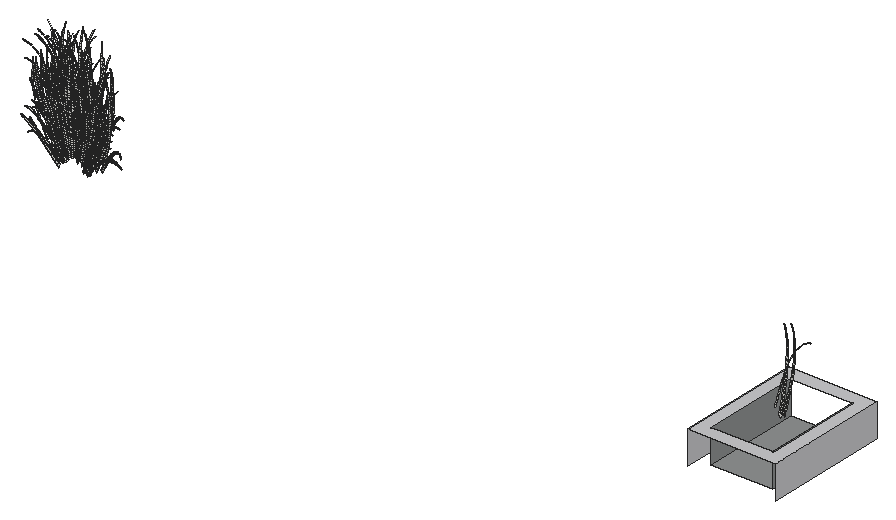
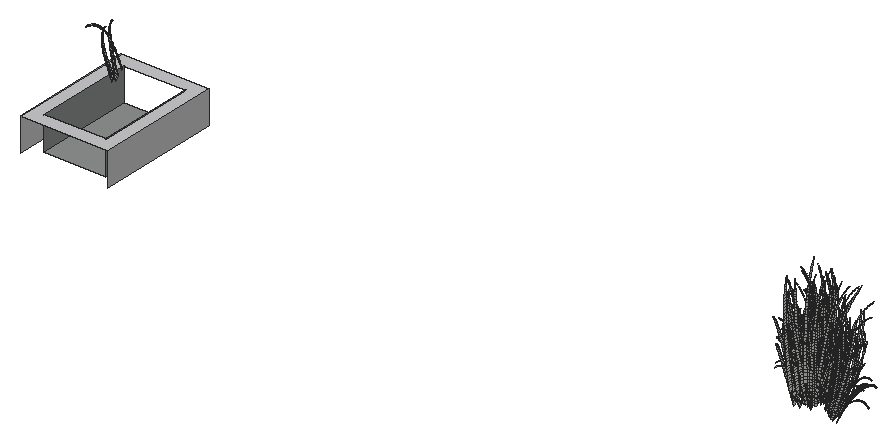
# SketchUp Ruby script. Lengths in inches.
U = 1.inch
M = Sketchup.active_model
def pt(a) = Geom::Point3d.new(a.map { |v| v * U })
def face(e, loops, mat)
  f = e.add_face(loops[0].map { |a| pt(a) })
  loops[1..].each { |l| e.add_face(l.map { |a| pt(a) }).erase! }
  f.material = f.back_material = mat if mat
  f
end
# faces: each face lists its corners as indices into pts; further lists are holes
def faces(e, pts, list, mat = nil) = list.each { |f| face(e, (f[0].is_a?(Array) ? f : [f]).map { |l| l.map { |i| pts[i] } }, mat) }
# xy, xz, yz: faces in a plane at the given z, y or x. An outline is a flat list of corners, or four numbers for a rectangle; further outlines are holes
def ring(l) = l.size == 4 ? [[l[0], l[1]], [l[2], l[1]], [l[2], l[3]], [l[0], l[3]]] : l.each_slice(2).to_a
def flat(e, list, mat, &to3) = list.each { |f| face(e, (f[0].is_a?(Array) ? f : [f]).map { |l| ring(l).map { |u, v| to3.(u, v) } }, mat) }
def xy(e, z, list, mat = nil) = flat(e, list, mat) { |x, y| [x, y, z] }
def xz(e, y, list, mat = nil) = flat(e, list, mat) { |x, z| [x, y, z] }
def yz(e, x, list, mat = nil) = flat(e, list, mat) { |y, z| [x, y, z] }
def lines(e, pts, list) = list.each { |a, b| e.add_line(pt(pts[a]), pt(pts[b])) }
# prism: a flat outline (further loops are holes) pulled along v
def prism(e, loops, v, mat = nil)
  f = face(e, loops, mat); d = Geom::Vector3d.new(v.map { |x| x * U })
  f.pushpull(f.normal.samedirection?(d) ? d.length : -d.length)
end
def box(e, o, s, mat = nil) = prism(e, [[o, [o[0] + s[0], o[1], o[2]], [o[0] + s[0], o[1] + s[1], o[2]], [o[0], o[1] + s[1], o[2]]]], [0, 0, s[2]], mat)
def at(x, y, z, deg = 0) = Geom::Transformation.translation(pt([x, y, z])) * Geom::Transformation.rotation(ORIGIN, Z_AXIS, deg.degrees)
def axes(o, x, y, z) = Geom::Transformation.new([*x, 0, *y, 0, *z, 0, *pt(o).to_a, 1])
def part(name) = M.definitions.add(name)
# library, detail: a bought-in or finely detailed component or shape, given as its bounding box
def library(name, o, s) = part(name).tap { |d| box(d.entities, o, s) }
def detail(e, o, s) = box(e.add_group.entities, o, s)
def put(e, d, t, mat = nil) = e.add_instance(d, t).tap { |i| i.material = mat if mat }
def group(e, t, mat = nil) = e.add_group.tap { |g| g.transformation = t; g.material = mat if mat }.entities
root = M.entities
M.materials.add("[Blacktop Old 02]").color = [143, 145, 145]
M.materials.add("[Polished Concrete New]").color = [200, 200, 203]
c1 = part("fur_instance\#8")
p = [[-0.25,1.49,0.03],[0.25,-1.49,-0.03],[0.44,-1.47,1.51],[-0.05,1.47,1.57],[0.65,-1.44,3.05],[0.16,1.45,3.11],
  [0.86,-1.42,4.59],[0.38,1.44,4.65],[1.1,-1.39,6.13],[0.62,1.43,6.18],[1.34,-1.35,7.66],[0.875,1.42,7.72],
  [1.6,-1.32,9.19],[1.14,1.41,9.25],[1.88,-1.28,10.72],[1.43,1.41,10.78],[2.18,-1.24,12.25],[1.73,1.41,12.3],
  [2.49,-1.19,13.77],[2.05,1.41,13.82],[2.83,-1.15,15.29],[2.4,1.41,15.34],[3.18,-1.09,16.8],[2.76,1.42,16.85],
  [3.56,-1.03,18.31],[3.14,1.43,18.35],[3.96,-0.97,19.81],[3.55,1.44,19.85],[4.38,-0.91,21.3],[3.99,1.46,21.35],
  [4.84,-0.83,22.78],[4.45,1.48,22.83],[5.32,-0.76,24.26],[4.93,1.51,24.31],[5.82,-0.67,25.73],[5.45,1.54,25.77],
  [6.36,-0.59,27.18],[6,1.57,27.23],[6.93,-0.49,28.625],[6.58,1.61,28.67],[7.54,-0.39,30.05],[7.19,1.66,30.1],
  [8.18,-0.28,31.47],[7.84,1.71,31.51],[8.85,-0.16,32.86],[8.53,1.77,32.9],[9.57,-0.04,34.24],[9.25,1.83,34.27],
  [10.32,0.09,35.59],[10.02,1.9,35.625],[11.12,0.23,36.92],[10.82,1.97,36.95],[11.95,0.38,38.22],[11.67,2.06,38.25],
  [12.84,0.54,39.49],[12.57,2.14,39.52],[13.76,0.71,40.73],[13.51,2.24,40.76],[14.73,0.89,41.93],[14.49,2.34,41.95],
  [15.75,1.08,43.09],[15.52,2.45,43.11],[16.82,1.28,44.2],[16.6,2.5625,44.23],[17.93,1.5,45.27],[17.73,2.68,45.29],
  [19.08,1.73,46.28],[18.9,2.81,46.3],[20.29,1.97,47.24],[20.125,2.93,47.26],[21.53,2.22,48.13],[21.39,3.0625,48.15],
  [22.82,2.5,48.96],[22.7,3.1875,48.98],[24.14,2.8125,49.72],[24.06,3.3,49.73],[25.48,3.27,50.41]]
faces(c1.entities,p,[[0,1,2,3],[3,2,4,5],[5,4,6,7],[7,6,8,9],[9,8,10,11],[11,10,12,13],[13,12,14,15],[15,14,16,17],
  [17,16,18,19],[19,18,20,21],[21,20,22,23],[23,22,24,25],[25,24,26,27],[27,26,28,29],[29,28,30,31],[31,30,32,33],
  [33,32,34,35],[35,34,36,37],[37,36,38,39],[39,38,40,41],[41,40,42,43],[43,42,44,45],[45,44,46,47],[47,46,48,49],
  [49,48,50,51],[51,50,52,53],[53,52,54,55],[55,54,56,57],[57,56,58,59],[59,58,60,61],[61,60,62,63],[63,62,64,65],
  [65,64,66,67],[67,66,68,69],[69,68,70,71],[71,70,72,73],[73,72,74,75],[75,74,76]])
xy(root,0,[[419.51,51.02,438.8125,82.15]],"[Blacktop Old 02]")
xy(root,10.375,[[[415.52,47.02,442.8125,86.15],[419.51,51.02,438.8125,82.15]]],"[Polished Concrete New]")
yz(root,415.52,[[47.02,0,86.15,10.375]],"[Polished Concrete New]")
yz(root,419.51,[[51.02,0,82.15,10.375]],"[Blacktop Old 02]")
yz(root,438.8125,[[51.02,0,82.15,10.375]],"[Blacktop Old 02]")
yz(root,442.8125,[[47.02,0,86.15,10.375]],"[Polished Concrete New]")
put(root,c1,axes([204.53,65.8125,2.49],[-0.13594,0.15084,-0.11164],[-0.0609,-0.07291,-0.33491],[-0.13519,-0.09407,0.27953]))
put(root,c1,axes([202.25,69.58,2.69],[0.13391,-0.00422,0.37894],[-0.02725,0.21287,-0.08205],[-0.17659,-0.01268,0.31548]))
put(root,c1,axes([204.92,66.53,3.77],[-0.14992,0.10635,-0.20855],[-0.03569,-0.13875,-0.18978],[-0.12006,-0.06524,0.33426]))
put(root,c1,axes([204.92,67.96,3.64],[-0.13947,0.07457,-0.26376],[-0.03048,-0.16347,-0.05841],[-0.12421,-0.01975,0.3263]))
put(root,c1,axes([204.95,66.7,2.23],[-0.11214,0.07357,-0.29467],[-0.00419,-0.1506,-0.10442],[-0.13991,-0.03543,0.25192]))
put(root,c1,axes([204.01,70.26,10.22],[-0.16722,-0.14584,-0.14657],[0.18274,-0.19209,0.09427],[-0.0816,-0.06233,0.55718]))
put(root,c1,axes([202.55,71.21,3.75],[0.10956,-0.18152,0.25882],[0.13509,0.11782,0.19082],[-0.14519,0.00192,0.39222]))
put(root,c1,axes([203.54,69.17,3.12],[0.07012,-0.18381,0.20265],[0.10518,0.07075,0.29594],[-0.16336,-0.01173,0.29184]))
put(root,c1,axes([203.42,66.95,2.47],[0.11177,0.01694,0.37048],[-0.08915,0.18926,-0.03147],[-0.15727,-0.07147,0.29687]))
put(root,c1,axes([203.95,67.58,2.98],[0.07273,0.09595,0.27862],[-0.10249,0.16133,-0.212],[-0.15668,-0.03967,0.28211]))
put(root,c1,axes([202.46,68.47,3.74],[0.16226,-0.13696,0.26442],[0.06401,0.16282,0.19515],[-0.14822,-0.05035,0.39313]))
put(root,c1,axes([205.3,68.57,8.76],[-0.19486,-0.07064,-0.15993],[0.11436,-0.20339,0.01183],[-0.07048,-0.06892,0.50496]))
put(root,c1,axes([205.51,65.35,1.82],[-0.09839,0.14314,-0.01192],[-0.08354,-0.02419,-0.30566],[-0.11714,-0.08151,0.24221]))
put(root,c1,axes([204.9,68.2,2.32],[-0.01321,-0.17005,0.06481],[0.1141,-0.02557,0.30569],[-0.13946,0.01456,0.25678]))
put(root,c1,axes([206.01,69.16,6.58],[-0.18243,0.01895,-0.19563],[-0.00133,-0.1948,0.08688],[-0.09334,0.00298,0.40574]))
put(root,c1,axes([205.88,67.88,4.63],[-0.16023,0.03354,-0.19126],[-0.00898,-0.17162,0.02853],[-0.08895,-0.01176,0.36236]))
put(root,c1,axes([205.84,66.625,5.96],[-0.1494,0.14445,-0.05993],[-0.10862,-0.10225,-0.21391],[-0.08642,-0.08137,0.39881]))
put(root,c1,axes([203.33,68.125,4.63],[0.16036,-0.12824,0.26431],[0.05712,0.1633,0.18167],[-0.14465,-0.04914,0.38366]))
put(root,c1,axes([203.74,68.18,3.85],[0.12489,0.06673,0.27563],[-0.09958,0.18305,-0.12082],[-0.13573,-0.04611,0.36]))
put(root,c1,axes([206.14,66.73,4.46],[-0.15052,-0.00251,-0.18515],[0.03159,-0.16716,0.03488],[-0.08794,-0.02622,0.34898]))
put(root,c1,axes([206.22,68.06,3.03],[-0.10384,0.1021,-0.23208],[-0.0841,-0.12138,-0.04288],[-0.10059,0.0191,0.29067]))
put(root,c1,axes([205.87,68.69,5.18],[-0.10618,-0.13262,-0.04878],[0.13367,-0.1263,0.19427],[-0.08735,0.00279,0.37967]))
put(root,c1,axes([204.71,68.18,1.81],[0.10833,0.05099,0.24664],[-0.03776,0.16401,-0.19126],[-0.1393,0.01454,0.25647]))
put(root,c1,axes([205.83,70.78,11.4],[-0.09372,-0.20637,-0.07363],[0.22677,-0.12712,0.15354],[-0.08199,-0.04812,0.55353]))
put(root,c1,axes([204.25,69.19,4.28],[0.15491,-0.05585,0.29054],[0.02871,0.18789,-0.02061],[-0.13151,0.00174,0.35528]))
put(root,c1,axes([206.86,67.92,5.72],[-0.13836,0.10656,-0.19014],[-0.08729,-0.13946,-0.02631],[-0.08371,0.00267,0.36384]))
put(root,c1,axes([205.74,66.87,3.52],[0.03066,0.14936,0.05869],[-0.12804,0.07175,-0.24213],[-0.11455,-0.01821,0.30092]))
put(root,c1,axes([206.11,66.9375,7.41],[-0.03053,0.18634,0.11663],[-0.19498,0.03215,-0.20672],[-0.09234,-0.08694,0.42611]))
put(root,c1,axes([206.36,66.09,6],[-0.076,0.1669,0.09562],[-0.17144,-0.01335,-0.19918],[-0.07397,-0.09509,0.39348]))
put(root,c1,axes([206.68,67.9,6.33],[-0.14595,-0.08896,-0.08701],[0.11069,-0.159,0.08949],[-0.05969,-0.02587,0.41282]))
put(root,c1,axes([206.68,66.87,6.51],[-0.13003,0.1505,-0.04051],[-0.13515,-0.09639,-0.12681],[-0.0585,-0.05721,0.41915]))
put(root,c1,axes([206.67,69.73,10.31],[-0.20007,-0.1011,-0.05198],[0.13259,-0.20105,0.02025],[-0.03025,-0.05245,0.53866]))
put(root,c1,axes([207.18,69.61,11.42],[-0.23914,-0.05106,-0.06078],[0.08551,-0.22855,-0.0252],[-0.02809,-0.06875,0.5682]))
put(root,c1,axes([205.61,67.93,1.8125],[0.06974,-0.11239,0.27242],[0.09117,0.10684,0.0892],[-0.12045,0.03482,0.23783]))
put(root,c1,axes([204.79,69.49,3.4],[0.12819,-0.10555,0.27193],[0.08655,0.15023,0.02614],[-0.11644,0.02211,0.33646]))
put(root,c1,axes([205.78,66.64,2.11],[0.09888,-0.02928,0.28041],[-0.00291,0.15131,-0.01175],[-0.12783,-0.00918,0.22836]))
put(root,c1,axes([206.3,68.41,3.74],[-0.01787,-0.16163,0.13786],[0.14541,-0.01364,0.20157],[-0.09392,0.03632,0.30351]))
put(root,c1,axes([207.22,66.9,5.53],[-0.15295,0.08658,-0.10984],[-0.06653,-0.14152,-0.02919],[-0.05435,-0.02356,0.3759]))
put(root,c1,axes([206.88,68.36,3.76],[-0.08732,-0.12975,0.07004],[0.12156,-0.08169,0.22443],[-0.07712,0.04857,0.29461]))
put(root,c1,axes([207.7,69.47,11.48],[-0.24023,0.10194,-0.01182],[-0.08393,-0.20819,-0.06775],[-0.02132,-0.07588,0.56748]))
put(root,c1,axes([205.42,66.95,3.46],[0.13512,-0.04534,0.25565],[0.00767,0.16418,0.01521],[-0.11775,-0.01872,0.30933]))
put(root,c1,axes([207.58,66.88,5.49],[-0.16155,0.04363,-0.11105],[-0.02173,-0.15615,0.00187],[-0.05311,-0.02302,0.36735]))
put(root,c1,axes([207.49,68.14,5.39],[-0.13763,-0.08778,-0.02445],[0.09224,-0.14199,0.18002],[-0.06167,0.02548,0.35158]))
put(root,c1,axes([207.18,67.91,9.83],[-0.11071,0.19643,0.08485],[-0.20741,-0.05916,-0.14436],[-0.04649,-0.10158,0.50968]))
put(root,c1,axes([205.5,67.375,5.75],[0.12398,0.09622,0.18511],[-0.12468,0.16008,-0.11198],[-0.09878,-0.04719,0.39625]))
put(root,c1,axes([207.82,67.29,6.31],[-0.15275,-0.06369,-0.07605],[0.08272,-0.1606,0.08732],[-0.05298,-0.01559,0.38969]))
put(root,c1,axes([207.65,66.44,5.47],[-0.12167,0.12231,-0.08026],[-0.10576,-0.10199,-0.07795],[-0.05387,-0.03162,0.36369]))
put(root,c1,axes([206.15,67.73,5.89],[0.1073,0.11537,0.13468],[-0.12896,0.14123,-0.15523],[-0.09593,-0.0286,0.38067]))
put(root,c1,axes([208.05,66.98,5.32],[-0.15222,0.06371,-0.10078],[-0.04912,-0.14483,0.02613],[-0.04368,-0.00705,0.35627]))
put(root,c1,axes([208.2,66.57,7.14],[-0.18454,0.07316,-0.01839],[-0.05778,-0.16138,-0.04792],[-0.01906,-0.05522,0.43193]))
put(root,c1,axes([206.91,71.5625,10.07],[-0.03022,-0.22611,0.09029],[0.23429,-0.05028,0.11994],[-0.05481,-0.00145,0.5217]))
put(root,c1,axes([206.39,65.9,6.21],[0.08886,0.11953,0.22309],[-0.17307,0.12603,-0.0526],[-0.07674,-0.09865,0.40821]))
put(root,c1,axes([208.3125,69.69,10.62],[-0.19122,-0.11806,-0.01455],[0.14538,-0.19433,0.04316],[-0.02276,-0.03764,0.53822]))
put(root,c1,axes([207.32,68.76,6.79],[-0.07059,-0.16734,0.04684],[0.17777,-0.08469,0.11217],[-0.04438,-0.00118,0.42241]))
put(root,c1,axes([208.41,67.4,6.18],[-0.1632,-0.04584,-0.02491],[0.06111,-0.16287,0.10545],[-0.03205,0.00396,0.38155]))
put(root,c1,axes([207.63,67.78,5.81],[-0.07809,-0.14325,0.0107],[0.15359,-0.09235,0.11164],[-0.04706,-0.00759,0.38378]))
put(root,c1,axes([208.48,68.24,7.07],[-0.18597,0.0618,-0.02273],[-0.04748,-0.17087,0.02426],[-0.01189,-0.02692,0.4292]))
put(root,c1,axes([206.75,67.35,3.28],[0.12505,0.02128,0.17693],[-0.02026,0.14885,-0.13694],[-0.09536,0.01811,0.27556]))
put(root,c1,axes([204.86,70.37,10.29],[0.23978,-0.07082,0.15768],[0.03022,0.22441,0.06362],[-0.07961,-0.06081,0.54364]))
put(root,c1,axes([207.61,68.31,8.43],[-0.04674,0.1979,-0.00041],[-0.20698,-0.02041,-0.04932],[-0.02674,-0.04637,0.47621]))
put(root,c1,axes([205.27,68.09,9.79],[0.21026,0.07749,0.17035],[-0.13208,0.20951,0.0486],[-0.06062,-0.09852,0.54406]))
put(root,c1,axes([205.62,69.1,7.84],[0.19711,0.03834,0.13931],[-0.07116,0.20343,-0.04176],[-0.07003,-0.0411,0.47276]))
put(root,c1,axes([206.98,67.91,4.64],[0.08378,-0.14307,0.16626],[0.13275,0.07958,0.06416],[-0.07048,0.0146,0.34149]))
put(root,c1,axes([208.77,65.47,5.33],[-0.14611,0.07417,-0.01085],[-0.0636,-0.12579,-0.04088],[-0.01571,-0.04551,0.35595]))
put(root,c1,axes([208.28,65.52,5.27],[-0.03907,0.14419,0.04289],[-0.15068,-0.00691,-0.10234],[-0.04404,-0.05511,0.34471]))
put(root,c1,axes([209.09,66.39,7.37],[-0.18895,0.06999,0.02245],[-0.05996,-0.16418,-0.04942],[-0.00199,-0.06326,0.44045]))
put(root,c1,axes([208.12,68.33,9.8125],[-0.07149,0.20688,0.05021],[-0.22153,-0.04139,-0.03916],[-0.01557,-0.07173,0.51835]))
put(root,c1,axes([208.72,67.78,4.4],[-0.12985,-0.07677,0.07158],[0.09092,-0.12597,0.14453],[-0.01646,0.03757,0.31821]))
put(root,c1,axes([208.21,66.36,5.48],[0.0007,0.15498,-0.03624],[-0.15701,0.01919,-0.0982],[-0.04789,-0.01409,0.35225]))
put(root,c1,axes([206,69.85,8.71],[0.21533,-0.00022,0.14201],[-0.02985,0.21622,-0.04212],[-0.07083,-0.0307,0.48991]))
put(root,c1,axes([208.125,69.9,6.69],[-0.05762,-0.17661,0.09378],[0.18885,-0.07013,0.07584],[-0.02585,0.00825,0.42914]))
put(root,c1,axes([208.84,66.12,6.67],[-0.11204,0.14362,0.03398],[-0.14775,-0.08605,-0.03808],[-0.00899,-0.05843,0.41243]))
put(root,c1,axes([207.78,66.88,5.72],[0.07256,0.13813,0.01061],[-0.14853,0.08916,-0.10968],[-0.05042,-0.01484,0.37084]))
put(root,c1,axes([209.64,68.28,7.88],[-0.20122,0.04978,0.02765],[-0.03696,-0.18587,0.02525],[0.00919,-0.0352,0.4569]))
put(root,c1,axes([208.44,69.16,7.99],[-0.07053,-0.17965,0.10788],[0.19435,-0.08267,0.06265],[-0.01549,0.01046,0.44704]))
put(root,c1,axes([209.05,67,5.46],[-0.12044,0.11617,-0.06507],[-0.11184,-0.10532,0.07409],[-0.00291,0.00808,0.35453]))
put(root,c1,axes([207.45,66.82,6.85],[0.1306,0.09776,0.12408],[-0.13059,0.14634,-0.04229],[-0.05761,-0.05634,0.41276]))
put(root,c1,axes([209.31,67,5.7],[-0.14146,0.09732,-0.03277],[-0.08974,-0.12702,0.09515],[0.00654,0.00629,0.36155]))
put(root,c1,axes([208.625,66.14,7.21],[-0.02865,0.1632,0.13083],[-0.19416,0.00105,-0.04665],[-0.01776,-0.09378,0.4187]))
put(root,c1,axes([206.58,68.21,9.33],[0.21896,0.00722,0.14738],[-0.05367,0.20894,0.06409],[-0.06377,-0.07981,0.49923]))
put(root,c1,axes([208.51,66.79,5.79],[-0.005,0.15882,-0.01867],[-0.16818,0.01184,-0.02587],[-0.01594,-0.02637,0.37698]))
put(root,c1,axes([209.49,68.37,4.09],[-0.15178,-0.03817,0.09021],[0.05761,-0.14672,0.13772],[0.01323,0.03497,0.32535]))
put(root,c1,axes([209.45,68.04,4.65],[-0.14817,-0.05096,0.10268],[0.07099,-0.14472,0.13123],[0.01339,0.03539,0.32926]))
put(root,c1,axes([209.01,65.7,5.82],[-0.04364,0.1509,0.04181],[-0.16335,-0.02313,-0.02043],[-0.0082,-0.05328,0.37608]))
put(root,c1,axes([207.61,66.81,6.55],[0.16328,0.03799,0.12354],[-0.06943,0.16853,-0.0179],[-0.05845,-0.04464,0.39911]))
put(root,c1,axes([209.2,68.17,5.49],[-0.0829,-0.13844,0.09301],[0.15279,-0.09132,0.04718],[-0.00308,0.00854,0.37496]))
put(root,c1,axes([207.75,68.7,6.83],[0.11915,-0.15444,0.11959],[0.14734,0.10329,0.01409],[-0.04397,-0.00116,0.41847]))
put(root,c1,axes([207.22,68.36,6.46],[0.18469,-0.02182,0.1026],[0.00322,0.18141,-0.06268],[-0.05045,-0.00814,0.41143]))
put(root,c1,axes([209.33,67.02,8.61],[-0.06667,0.19226,0.05915],[-0.20819,-0.04319,-0.00198],[0.00188,-0.06909,0.48578]))
put(root,c1,axes([209.45,68.83,6.34],[-0.10911,-0.1372,0.1051],[0.15387,-0.1168,0.04236],[0.00736,0.00708,0.40712]))
put(root,c1,axes([208.07,70.77,5.5],[0.05449,-0.17808,0.19773],[0.18828,0.03949,-0.026],[-0.02035,0.04645,0.39347]))
put(root,c1,axes([207.875,66.2,5.34],[0.15146,0.01629,0.10652],[-0.04117,0.15418,-0.02273],[-0.05245,-0.03078,0.35407]))
put(root,c1,axes([208.59,69.19,6.84],[0.00836,-0.18662,0.11674],[0.19508,-0.00753,0.01588],[-0.01463,0.00988,0.4222]))
put(root,c1,axes([207.5625,68.6,8.21],[0.12224,-0.1724,0.03147],[0.17004,0.09672,0.03094],[-0.02457,-0.03858,0.46994]))
put(root,c1,axes([208.79,71.77,9.61],[-0.01914,-0.22341,0.14227],[0.23668,-0.03758,0.00754],[-0.0042,0.01167,0.5122]))
put(root,c1,axes([209.73,65.51,5.34],[-0.08483,0.12977,0.03637],[-0.13576,-0.06868,0.01436],[0.01015,-0.0438,0.35695]))
put(root,c1,axes([207.98,66.92,7.01],[0.13112,0.1119,0.04642],[-0.13781,0.13647,-0.01148],[-0.02271,-0.04835,0.42618]))
put(root,c1,axes([207.09,67.25,9.36],[0.22597,0.02863,0.10796],[-0.07525,0.20019,0.13019],[-0.03474,-0.10937,0.51158]))
put(root,c1,axes([209.94,70.6,7.58],[-0.12335,-0.15584,0.12717],[0.17408,-0.13265,0.02266],[0.01997,0.00343,0.46197]))
put(root,c1,axes([209.21,68.51,7.9375],[-0.03248,-0.18789,0.03246],[0.20264,-0.04691,-0.01246],[0.00277,-0.0305,0.45814]))
put(root,c1,axes([208.61,70.71,5.47],[0.06236,-0.17527,0.19539],[0.18475,0.04701,-0.03446],[-0.02024,0.04621,0.39144]))
put(root,c1,axes([206.73,70.18,11.4],[0.24246,-0.09581,0.04741],[0.07374,0.21618,0.03906],[-0.03158,-0.05994,0.56838]))
put(root,c1,axes([208.96,69.22,8.11],[0.00458,-0.19714,0.03462],[0.20895,-0.01368,-0.00104],[-0.00501,-0.02872,0.46671]))
put(root,c1,axes([208.42,66.2,8.97],[0.08928,0.17665,0.16183],[-0.22737,0.09539,0.05927],[-0.00818,-0.11915,0.51927]))
put(root,c1,axes([207.9,68.33,5.63],[0.167,0.03821,0.03014],[-0.05354,0.16593,-0.1048],[-0.03226,0.00399,0.38398]))
put(root,c1,axes([210.21,67.23,4.97],[-0.11227,0.12169,-0.01571],[-0.11695,-0.0983,0.09825],[0.0234,-0.00238,0.35291]))
put(root,c1,axes([209.68,68.5,10.47],[-0.01737,0.2214,0.05487],[-0.24332,0.00145,0.03189],[0.01003,-0.07326,0.54284]))
put(root,c1,axes([209.4375,65.79,7.44],[-0.01068,0.1751,0.14296],[-0.21108,0.00073,0.04004],[0.01667,-0.10172,0.45077]))
put(root,c1,axes([209.92,68.3,8.15],[-0.03706,0.19452,0.0025],[-0.2058,-0.02021,0.04233],[0.01369,-0.04269,0.4672]))
put(root,c1,axes([209.44,67.62,8.14],[0.00321,0.19067,0.02092],[-0.20749,0.01649,0.04397],[0.01444,-0.0534,0.46311]))
put(root,c1,axes([209.28,66.97,6.03],[0.0444,0.15353,-0.02873],[-0.16709,0.05572,0.00025],[-0.00083,-0.02443,0.38596]))
put(root,c1,axes([207.91,67.77,7.43],[0.19137,0.02245,0.03812],[-0.04546,0.1843,-0.01629],[-0.02307,-0.03624,0.44138]))
put(root,c1,axes([208.93,69.2,9.32],[0.0752,-0.20516,0.02464],[0.21175,0.0536,-0.02901],[0.00304,-0.03339,0.50163]))
put(root,c1,axes([208.76,70.36,5.36],[0.1059,-0.15637,0.15831],[0.16025,0.08485,-0.11228],[-0.00207,0.04487,0.3837]))
put(root,c1,axes([211.15,69.14,9.93],[-0.20879,-0.09834,0.1321],[0.10662,-0.20129,-0.08744],[0.06463,-0.06137,0.52082]))
put(root,c1,axes([209.47,67.43,5.97],[0.04623,0.15623,-0.10375],[-0.16763,0.05842,0.01792],[0.01628,0.0028,0.37652]))
put(root,c1,axes([208.76,66.62,5.85],[0.15712,0.04243,0.01115],[-0.06087,0.1538,-0.0283],[-0.01337,-0.02475,0.37716]))
put(root,c1,axes([209.95,67.09,5.42],[-0.02615,-0.15514,0.08978],[0.1636,-0.03862,-0.04775],[0.02391,-0.00243,0.36067]))
put(root,c1,axes([208.65,68.37,5.37],[0.17226,-0.02677,0.04434],[0.01787,0.15893,-0.17055],[-0.01798,0.04104,0.34767]))
put(root,c1,axes([208.55,69.57,7.86],[0.17834,-0.11625,0.08266],[0.1071,0.16149,-0.09447],[-0.01558,0.01053,0.44981]))
put(root,c1,axes([211.33,67.0625,7],[-0.15292,0.11854,0.12624],[-0.12574,-0.14279,0.04956],[0.05301,-0.06232,0.4383]))
put(root,c1,axes([210.57,68.91,4.93],[-0.09023,-0.13424,0.18354],[0.14991,-0.10591,-0.00994],[0.04513,0.02354,0.36032]))
put(root,c1,axes([210.12,66.69,5.33],[0.01188,0.15545,-0.07184],[-0.16156,0.0237,0.07132],[0.03067,-0.00873,0.35494]))
put(root,c1,axes([210.0625,65.76,5.75],[-0.00201,0.1516,0.05729],[-0.16575,-0.0022,0.09935],[0.04109,-0.06021,0.3647]))
put(root,c1,axes([211.45,67.33,4.33],[-0.15312,0.05179,0.12153],[-0.03636,-0.15379,0.12597],[0.06399,-0.0008,0.33763]))
put(root,c1,axes([209.48,66.54,5.63],[0.13491,0.07893,-0.02845],[-0.09527,0.13412,-0.00523],[0.005,-0.02625,0.36875]))
put(root,c1,axes([210.19,69.04,4.84],[0.00974,-0.16765,0.16266],[0.17627,-0.01134,-0.08044],[0.03031,0.03221,0.35757]))
put(root,c1,axes([211.03,66.65,5.01],[-0.12808,-0.08127,0.17105],[0.08472,-0.13879,-0.03962],[0.07069,-0.01437,0.33524]))
put(root,c1,axes([210.13,72.16,11.75],[-0.01557,-0.2472,0.11257],[0.25666,-0.03446,-0.11464],[0.04868,-0.01385,0.56337]))
put(root,c1,axes([209.36,68.8,11.2],[0.1638,0.16225,0.02835],[-0.19372,0.16204,0.06129],[0.00656,-0.07857,0.56406]))
put(root,c1,axes([209.86,67.81,4.25],[0.06075,-0.14439,0.11282],[0.14535,0.04045,-0.11615],[0.02704,0.02874,0.31908]))
put(root,c1,axes([210.27,67.84,9.05],[0.00546,0.20018,0.07075],[-0.21886,0.00452,0.13393],[0.05427,-0.07952,0.48166]))
put(root,c1,axes([209.32,69.05,8.9],[0.1489,-0.1631,0.00196],[0.16131,0.12724,-0.0384],[0.00665,-0.0349,0.49014]))
put(root,c1,axes([211.88,68.03,5.81],[-0.17727,-0.00884,0.19718],[0.01815,-0.18643,0.05134],[0.08203,-0.01667,0.38902]))
put(root,c1,axes([208.84,68.81,10.45],[0.24085,-0.01288,-0.01594],[-0.00713,0.21681,0.06326],[0.00207,-0.07616,0.53545]))
put(root,c1,axes([211.97,68.4,7.44],[-0.19467,0.01004,0.22404],[-0.00781,-0.20399,0.04036],[0.09618,-0.03688,0.42982]))
put(root,c1,axes([208.84,69.48,11.5625],[0.24462,0.04853,-0.00958],[-0.07419,0.22591,0.06737],[0.00661,-0.07917,0.56836]))
put(root,c1,axes([209.61,67.41,5.75],[0.16085,-0.07091,-0.00868],[0.05991,0.14859,-0.10356],[0.01607,0.00276,0.37166]))
put(root,c1,axes([211.58,66.49,4.31],[-0.09933,0.11915,0.09682],[-0.11277,-0.10305,0.14649],[0.07419,-0.02845,0.33155]))
put(root,c1,axes([210.33,65.87,7.53],[0.1142,0.15271,0.07486],[-0.18421,0.10064,0.13224],[0.02836,-0.10071,0.46512]))
put(root,c1,axes([210.75,66.91,4.26],[0.01848,-0.15029,0.09797],[0.14831,0.00119,-0.12824],[0.05045,0.01072,0.31409]))
put(root,c1,axes([209.47,67.96,8.99],[0.21441,0.03504,-0.02755],[-0.05444,0.19871,0.04867],[0.01191,-0.06374,0.49276]))
put(root,c1,axes([209.98,66.59,5.26],[0.15483,0.02452,-0.08835],[-0.03742,0.15266,-0.04583],[0.03016,-0.00858,0.34899]))
put(root,c1,axes([210.47,66.39,4.93],[0.12172,0.08749,-0.09823],[-0.09805,0.12464,0.01693],[0.03543,-0.01566,0.34464]))
put(root,c1,axes([212.01,70.26,6.49],[-0.10531,-0.16415,0.20039],[0.16955,-0.12413,-0.09552],[0.08116,-0.00102,0.4282]))
put(root,c1,axes([210.02,67.3,6.65],[0.15584,0.0797,-0.11547],[-0.0923,0.15744,0.00315],[0.04105,-0.01815,0.39937]))
put(root,c1,axes([213.06,68.26,7.57],[-0.20296,0.04396,0.25147],[-0.06114,-0.20583,-0.00189],[0.10319,-0.08007,0.46398]))
put(root,c1,axes([211.79,66.9,5.41],[-0.05241,0.16147,0.07727],[-0.15892,-0.06034,0.18232],[0.08415,-0.0479,0.3696]))
put(root,c1,axes([210.74,66.85,5.91],[0.10935,0.12723,-0.0806],[-0.13524,0.11022,0.08276],[0.04716,-0.03593,0.38648]))
put(root,c1,axes([212.25,66.15,3.65],[-0.13363,0.01209,0.24348],[-0.02341,-0.15821,0.02454],[0.10585,-0.04288,0.29749]))
put(root,c1,axes([210.95,65.54,4.49],[0.04868,0.13833,-0.04452],[-0.13249,0.04478,0.16098],[0.07098,-0.0404,0.31175]))
put(root,c1,axes([210.42,68.62,3.92],[0.15705,-0.06817,-0.01855],[0.04537,0.13415,-0.23216],[0.04015,0.05663,0.29621]))
put(root,c1,axes([211.52,66.96,3.72],[-0.0035,0.15221,-0.13037],[-0.13811,0.0204,0.18439],[0.08356,0.01425,0.28222]))
put(root,c1,axes([210.47,68.01,9.67],[0.18476,0.1259,-0.03463],[-0.14125,0.16417,0.15823],[0.05053,-0.09421,0.50755]))
put(root,c1,axes([212.53,67.04,4.53],[-0.105,0.10997,0.20265],[-0.1047,-0.1341,0.17455],[0.11569,-0.04687,0.32514]))
put(root,c1,axes([210.73,68.72,6.91],[0.18917,-0.06704,-0.06686],[0.05451,0.17895,-0.10326],[0.03727,-0.0106,0.43133]))
put(root,c1,axes([212.07,67.5,1.76],[-0.02967,-0.12807,0.22483],[0.11753,-0.07372,-0.14887],[0.10049,0.02798,0.22698]))
put(root,c1,axes([210.32,69.07,8.93],[0.21551,0.00607,-0.13742],[-0.0172,0.21045,-0.03067],[0.05502,-0.03283,0.47913]))
put(root,c1,axes([210.81,67.71,6.93],[0.18544,-0.04972,-0.1199],[0.04511,0.1779,-0.04118],[0.05175,-0.03943,0.42412]))
put(root,c1,axes([213.64,69.2,8.01],[-0.13857,0.17143,0.18015],[-0.17196,-0.14956,0.18932],[0.11106,-0.06322,0.48777]))
put(root,c1,axes([212.97,69.35,3.87],[-0.08271,-0.14836,0.25336],[0.14839,-0.11682,-0.11362],[0.10275,0.01753,0.34702]))
put(root,c1,axes([211.26,67.73,3.55],[0.1392,0.01865,-0.19659],[-0.04604,0.15192,-0.11441],[0.07206,0.03039,0.28637]))
put(root,c1,axes([210.91,69.6875,8.92],[0.2045,-0.09371,-0.11076],[0.08595,0.19464,-0.09275],[0.05645,-0.03369,0.4916]))
put(root,c1,axes([211.38,71.22,8.32],[0.13505,-0.18869,0.02697],[0.17317,0.11473,-0.23558],[0.07413,0.01575,0.4615]))
put(root,c1,axes([213.46,68.18,6.88],[-0.05009,0.1972,0.12811],[-0.20341,-0.06615,0.21296],[0.10198,-0.07913,0.45854]))
put(root,c1,axes([213.05,67.67,4.17],[-0.05226,0.17384,0.04608],[-0.14605,-0.06174,0.27189],[0.11826,-0.02606,0.33853]))
put(root,c1,axes([212.61,65.9375,2.1],[-0.0259,0.13847,0.08839],[-0.10293,-0.05886,0.26708],[0.12297,-0.03787,0.2304]))
put(root,c1,axes([211.51,67.41,6.72],[0.19428,0.00099,-0.13011],[-0.00447,0.1857,0.01775],[0.05358,-0.05088,0.43173]))
put(root,c1,axes([212.84,67.67,2.35],[-0.0586,-0.13145,0.25194],[0.10919,-0.10295,-0.16429],[0.12358,0.00811,0.25105]))
put(root,c1,axes([211.75,66.77,3.32],[0.11365,-0.08796,-0.13302],[0.06535,0.12495,-0.18142],[0.09174,-0.00314,0.27875]))
put(root,c1,axes([212.28,68.98,3.85],[0.12182,-0.13641,-0.05722],[0.10481,0.11532,-0.25636],[0.0972,0.01658,0.32827]))
put(root,c1,axes([212.03,68.15,4.4375],[0.15112,-0.07348,-0.15621],[0.04279,0.15836,-0.20373],[0.095,0.01621,0.32084]))
put(root,c1,axes([213.72,67.97,7.79],[0.03711,0.21617,0.09276],[-0.22705,0.0107,0.25479],[0.10293,-0.10542,0.49477]))
put(root,c1,axes([213.01,68.18,6.04],[0.10459,0.17012,-0.10766],[-0.16118,0.10117,0.20027],[0.09662,-0.055,0.42437]))
put(root,c1,axes([214.55,68.55,1.99],[-0.11534,0.10838,0.24896],[-0.07338,-0.1624,0.25205],[0.15325,-0.01897,0.29298]))
put(root,c1,axes([212.53,66.17,3.82],[0.13705,0.06092,-0.24143],[-0.03897,0.15511,0.08813],[0.11117,-0.04504,0.31244]))
put(root,c1,axes([214.24,69.52,4.5625],[-0.04683,-0.20253,0.13494],[0.1704,-0.05617,-0.28372],[0.13472,-0.02969,0.38568]))
put(root,c1,axes([212.8,66.62,3.24],[0.14053,0.00256,-0.25431],[0.0115,0.16488,-0.00221],[0.11001,-0.04457,0.30917]))
put(root,c1,axes([213.04,67.55,3.5625],[0.11573,-0.11352,-0.17299],[0.09518,0.13737,-0.20258],[0.11423,-0.02517,0.32701]))
put(root,c1,axes([213.875,65.75,2.08],[0.04443,0.16095,0.1082],[-0.13761,-0.02397,0.33152],[0.13789,-0.09974,0.2801]))
put(root,c1,axes([214.4,72.45,7.95],[0.03522,-0.24577,0.05534],[0.23308,0.0235,-0.26379],[0.10852,-0.02206,0.51462]))
put(root,c1,axes([214.21,66.45,2.2],[0.00679,0.17207,0.10989],[-0.13694,-0.04896,0.33579],[0.14998,-0.07528,0.28652]))
put(root,c1,axes([213.91,70.35,7.44],[0.1074,-0.20139,-0.09354],[0.19115,0.11076,-0.2385],[0.10824,-0.04151,0.48371]))
put(root,c1,axes([213.27,69.12,4.6],[0.15027,-0.10781,-0.18095],[0.0791,0.16599,-0.22838],[0.11882,-0.00407,0.36105]))
put(root,c1,axes([216.46,68.63,2.75],[-0.15284,0.01805,0.42901],[-0.06641,-0.2167,0.01891],[0.18229,-0.0915,0.34824]))
put(root,c1,axes([214.15,67.28,2.26],[0.12633,-0.01434,-0.33979],[0.03003,0.18353,-0.05493],[0.15045,-0.04633,0.28189]))
put(root,c1,axes([214.37,66.42,2.13],[0.13942,0.04831,-0.34302],[0.00816,0.17572,0.1089],[0.15278,-0.07668,0.29185]))
put(root,c1,axes([214.62,70.61,5.98],[0.12813,-0.17071,-0.17976],[0.14324,0.15198,-0.29056],[0.14651,-0.03228,0.41943]))
put(root,c1,axes([215.89,69.0625,2.38],[0.07286,-0.17069,-0.21842],[0.13329,0.1313,-0.33824],[0.176,-0.05419,0.32974]))
put(root,c1,axes([432.625,61.43,13.55],[-0.22222,0.12257,-0.08636],[-0.10729,-0.17964,0.33239],[0.02989,0.09528,0.43781]))
put(root,c1,axes([433,62.5,13.72],[-0.24957,0.08322,-0.01695],[-0.05226,-0.18613,0.43808],[0.0399,0.13857,0.37627]))
put(root,c1,axes([431.82,60.61,16.19],[0.16049,0.15534,-0.27829],[-0.19592,0.15388,-0.21201],[-0.00087,0.10351,0.44615]))
